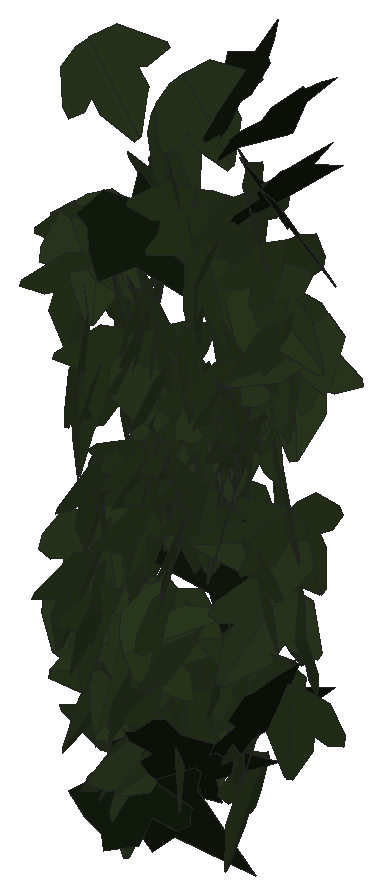
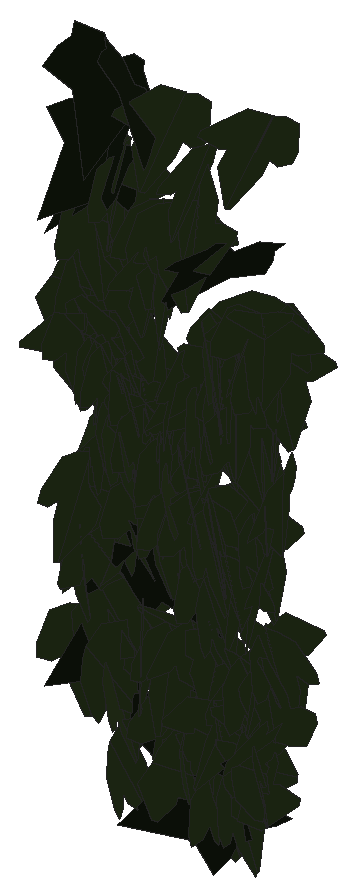
# SketchUp Ruby script. Lengths in inches.
U = 1.inch
M = Sketchup.active_model
def pt(a) = Geom::Point3d.new(a.map { |v| v * U })
def face(e, loops, mat)
  f = e.add_face(loops[0].map { |a| pt(a) })
  loops[1..].each { |l| e.add_face(l.map { |a| pt(a) }).erase! }
  f.material = f.back_material = mat if mat
  f
end
# faces: each face lists its corners as indices into pts; further lists are holes
def faces(e, pts, list, mat = nil) = list.each { |f| face(e, (f[0].is_a?(Array) ? f : [f]).map { |l| l.map { |i| pts[i] } }, mat) }
# xy, xz, yz: faces in a plane at the given z, y or x. An outline is a flat list of corners, or four numbers for a rectangle; further outlines are holes
def ring(l) = l.size == 4 ? [[l[0], l[1]], [l[2], l[1]], [l[2], l[3]], [l[0], l[3]]] : l.each_slice(2).to_a
def flat(e, list, mat, &to3) = list.each { |f| face(e, (f[0].is_a?(Array) ? f : [f]).map { |l| ring(l).map { |u, v| to3.(u, v) } }, mat) }
def xy(e, z, list, mat = nil) = flat(e, list, mat) { |x, y| [x, y, z] }
def xz(e, y, list, mat = nil) = flat(e, list, mat) { |x, z| [x, y, z] }
def yz(e, x, list, mat = nil) = flat(e, list, mat) { |y, z| [x, y, z] }
def lines(e, pts, list) = list.each { |a, b| e.add_line(pt(pts[a]), pt(pts[b])) }
# prism: a flat outline (further loops are holes) pulled along v
def prism(e, loops, v, mat = nil)
  f = face(e, loops, mat); d = Geom::Vector3d.new(v.map { |x| x * U })
  f.pushpull(f.normal.samedirection?(d) ? d.length : -d.length)
end
def box(e, o, s, mat = nil) = prism(e, [[o, [o[0] + s[0], o[1], o[2]], [o[0] + s[0], o[1] + s[1], o[2]], [o[0], o[1] + s[1], o[2]]]], [0, 0, s[2]], mat)
def at(x, y, z, deg = 0) = Geom::Transformation.translation(pt([x, y, z])) * Geom::Transformation.rotation(ORIGIN, Z_AXIS, deg.degrees)
def axes(o, x, y, z) = Geom::Transformation.new([*x, 0, *y, 0, *z, 0, *pt(o).to_a, 1])
def part(name) = M.definitions.add(name)
# library, detail: a bought-in or finely detailed component or shape, given as its bounding box
def library(name, o, s) = part(name).tap { |d| box(d.entities, o, s) }
def detail(e, o, s) = box(e.add_group.entities, o, s)
def put(e, d, t, mat = nil) = e.add_instance(d, t).tap { |i| i.material = mat if mat }
def group(e, t, mat = nil) = e.add_group.tap { |g| g.transformation = t; g.material = mat if mat }.entities
root = M.entities
M.materials.add("efeu1").color = [18, 25, 13]
M.materials.add("efeu2").color = [43, 57, 29]
c1 = part("ivyleaf_10")
p = [[0,0.5,-0.03],[-0.0625,2.02,-0.43],[-0.19,2.01,-0.46],[-0.54,1.05,-0.29],[-0.52,0.625,-0.18],[-0.83,0.76,-0.28],
  [-1.16,0.64,-0.33],[-1.15,0.33,-0.24],[-0.77,-0.39,0.02],[-0.3,-0.51,0.16],[0.04,-0.48,0.23],[-0.02,2.01,-0.4375],
  [-0.06,2.01,-0.43],[0.04,-0.49,0.23],[0.67,-0.49,0.14],[1.38,0.36,-0.2],[1.375,0.51,-0.24],[0.81,0.65,-0.19],
  [0.62,0.59,-0.15],[0.6,1.09,-0.28],[0.5,1.23,-0.31]]
faces(c1.entities,p,[[0,1,2,3,4,5,6,7,8,9,10],[11,12,0,13,14,15,16,17,18,19,20]],"efeu2")
c2 = part("ivyleaf_9")
p = [[1.54,2.16,1.25],[1.36,2.04,1.19],[-0.21,0.99,0.68],[-0.71,1.11,0.82],[-0.85,0.86,0.67],[-0.8,0.17,0.21],
  [-0.9,-0.01,0.1],[-0.67,-0.16,-0.02],[-0.08,-0.08,-0.05],[-0.03,-0.6,-0.4],[0.65,-0.88,-0.66],[0.83,-0.6,-0.49],
  [1.29,-0.42,-0.43],[1.8125,-0.07,-0.26],[1.21,0.44,0.15]]
faces(c2.entities,p,[[0,1,2,3,4,5,6,7,8,9,10,11,12,13,14]],"efeu1")
put(root,c1,axes([27.76,224.9,217.875],[0.32186,-0.37476,0.07721],[0.0469,-0.06149,-0.49398],[0.37975,0.32523,-0.00443]))
put(root,c1,axes([28.11,224.8,221.44],[-0.12731,-0.48235,-0.0336],[0.01522,0.03073,-0.49882],[0.48328,-0.12803,0.00686]))
put(root,c1,axes([27,224.88,220.98],[-0.45625,0.14667,0.14255],[0.12489,-0.0762,0.47812],[0.16197,0.47189,0.0329]))
put(root,c1,axes([27.65,224.8,218.9],[-0.48631,-0.11147,0.03275],[-0.01817,-0.06626,-0.49526],[0.11475,-0.48289,0.06039]))
put(root,c1,axes([26.05,224.64,219.4],[0.22603,-0.33922,-0.28955],[-0.06525,0.29596,-0.39768],[0.44119,0.21756,0.08952]))
put(root,c1,axes([26.27,224.625,222.59],[0.23053,0.39163,0.20853],[0.05646,0.20719,-0.45154],[-0.44008,0.23174,0.05131]))
put(root,c1,axes([26.78,224.75,219.79],[-0.43148,0.24494,-0.0619],[0.04889,-0.03924,-0.49605],[-0.24787,-0.43412,0.00992]))
put(root,c1,axes([27.88,224.69,219.13],[-0.44021,0.19722,0.13159],[-0.12185,0.04985,-0.48235],[-0.20338,-0.45675,0.00417]))
put(root,c2,axes([26.63,224.75,220.96],[0.11537,-0.37052,-0.31528],[0.09739,0.33505,-0.35813],[0.47666,0.02122,0.14948]))
put(root,c1,axes([26.12,224.875,217.59],[0.03942,-0.49822,0.01477],[-0.001,-0.0149,-0.49978],[0.49844,0.03937,-0.00217]))
put(root,c1,axes([26.59,225,214.24],[-0.12687,-0.45195,0.17217],[0.08725,-0.19647,-0.45143],[0.4757,-0.0845,0.12872]))
put(root,c1,axes([27.57,224.8125,221.0625],[-0.2853,-0.4062,-0.06001],[0.07845,0.0178,-0.49349],[0.40305,-0.291,0.05358]))
put(root,c1,axes([28.67,225.06,220.06],[0.1758,0.19948,-0.42344],[-0.3113,-0.28796,-0.2649],[-0.34955,0.35677,0.02295]))
put(root,c1,axes([25.92,224.91,219.86],[-0.25461,-0.41696,0.10639],[-0.0479,-0.09539,-0.48847],[0.42765,-0.25893,0.00863]))
put(root,c2,axes([26.96,224.72,214.59],[0.29944,0.22544,-0.33092],[0.26768,0.19461,0.3748],[0.29779,-0.40163,-0.00414]))
put(root,c1,axes([26.77,224.86,219.67],[0.15933,-0.47141,-0.04881],[-0.00204,0.05082,-0.49741],[0.47393,0.15871,0.01427]))
put(root,c1,axes([25.83,224.96,216.3125],[-0.01159,-0.48963,0.10065],[-0.01001,-0.10043,-0.48971],[0.49977,-0.01337,-0.00747]))
put(root,c1,axes([28.21,224.92,215.95],[-0.35874,-0.19812,0.28645],[-0.23915,-0.15883,-0.40936],[0.2532,-0.43072,0.0192]))
put(root,c1,axes([26.25,224.9,215.59],[0.48382,-0.12583,0.00893],[0.00832,-0.00348,-0.49992],[0.12587,0.48389,-0.00127]))
put(root,c1,axes([27.33,224.87,221.14],[-0.4268,-0.24203,0.09624],[-0.06571,-0.07872,-0.48937],[0.25204,-0.43038,0.03538]))
put(root,c1,axes([28.3125,224.92,216.72],[0.33343,0.27819,-0.24787],[-0.233,-0.10389,-0.43002],[-0.29075,0.40227,0.06036]))
put(root,c1,axes([28.45,224.9,220.91],[-0.19348,-0.46019,0.02807],[0.01283,-0.0358,-0.49855],[0.46087,-0.1922,0.02567]))
put(root,c1,axes([26.71,224.9,218.8],[0.30583,-0.03388,0.39411],[0.39529,0.00756,-0.30609],[0.01478,0.49879,0.03141]))
put(root,c1,axes([28.24,224.68,221.57],[-0.2867,0.36522,0.18552],[-0.14239,0.12348,-0.46312],[-0.3841,-0.31838,0.0332]))
put(root,c1,axes([28.24,224.81,220.44],[0.28634,0.09797,0.39801],[0.38316,0.1085,-0.30236],[-0.14561,0.47815,-0.01294]))
put(root,c2,axes([28.27,224.44,215.53],[0.17365,0.29767,0.36227],[0.16977,0.32019,-0.34447],[-0.43706,0.24264,0.01013]))
put(root,c1,axes([28.55,224.82,220.08],[-0.11985,-0.47617,-0.0943],[0.03761,0.08773,-0.4908],[0.48396,-0.12474,0.01479]))
put(root,c1,axes([27.95,224.87,219.72],[-0.39698,0.06214,-0.29757],[0.2846,-0.09601,-0.39973],[-0.10682,-0.48674,0.04086]))
put(root,c1,axes([26.8,224.75,215.83],[0.24577,-0.06021,-0.43124],[0.43309,0.08507,0.23495],[0.04508,-0.48902,0.09397]))
put(root,c2,axes([28.1875,224.79,221.81],[0.45684,-0.18155,-0.09128],[-0.08373,0.03647,-0.49159],[0.18515,0.46445,0.00291]))
put(root,c1,axes([26.62,224.97,219.1],[0.1077,-0.48462,0.05952],[0.02434,-0.05555,-0.49631],[0.48766,0.1098,0.01163]))
put(root,c1,axes([26.36,224.98,214.29],[0.05304,-0.49244,0.06846],[0.01417,-0.06732,-0.49524],[0.49698,0.05448,0.00682]))
put(root,c1,axes([28.42,224.96,217.51],[0.11904,0.03073,-0.48465],[-0.48181,-0.05495,-0.12182],[-0.06075,0.49602,0.01653]))
put(root,c1,axes([27.11,224.91,217.27],[0.22328,-0.44427,-0.05263],[-0.02908,0.04428,-0.49719],[0.44643,0.22508,-0.00606]))
put(root,c1,axes([25.92,224.9,220.45],[-0.37661,-0.1667,-0.2835],[0.31762,-0.07254,-0.37928],[0.08533,-0.46578,0.16053]))
put(root,c1,axes([27.66,224.58,220.39],[-0.04606,0.26392,0.42217],[-0.31505,0.31284,-0.22994],[-0.38552,-0.28719,0.13748]))
put(root,c2,axes([26.83,224.76,213.85],[-0.49327,-0.06522,0.04932],[0.04903,0.00549,0.49756],[-0.06544,0.4957,0.00098]))
put(root,c1,axes([27.625,224.78,220.59],[0.04077,0.49217,0.07813],[-0.03385,0.08094,-0.49224],[-0.49718,0.03485,0.03992]))
put(root,c1,axes([26.09,225.09,215.91],[-0.06239,-0.46204,0.18064],[0.03324,-0.18555,-0.46311],[0.49498,-0.04578,0.05387]))
put(root,c2,axes([28.47,224.58,222.67],[0.09332,0.47646,0.11949],[-0.01587,0.12449,-0.48399],[-0.49096,0.08654,0.03835]))
put(root,c1,axes([26.34,224.85,219.95],[-0.25046,0.43242,-0.01664],[-0.00683,-0.02317,-0.49942],[-0.43269,-0.24994,0.01752]))
put(root,c1,axes([26.91,225.2,214.72],[0.0959,-0.20544,0.44564],[0.34429,-0.29539,-0.21027],[0.34967,0.34719,0.08481]))
put(root,c1,axes([28.19,224.93,219.47],[-0.4104,0.16587,0.2325],[-0.2745,-0.11666,-0.4013],[-0.07887,-0.45703,0.18682]))
put(root,c1,axes([28.23,225.11,218.21],[0.16858,-0.24164,0.40397],[0.39421,-0.16204,-0.26143],[0.25726,0.40664,0.13588]))
put(root,c1,axes([28.02,224.9,217.2],[-0.40692,0.26497,-0.1192],[0.09256,-0.07623,-0.48541],[-0.27541,-0.41711,0.01299]))
put(root,c1,axes([26.98,224.98,216.14],[0.09407,0.46893,-0.14579],[-0.07354,-0.13331,-0.47626],[-0.48553,0.11105,0.04389]))
put(root,c1,axes([26.12,224.6875,216.05],[0.05681,-0.33327,-0.36838],[-0.02077,0.36887,-0.33691],[0.49633,0.05358,0.02806]))
put(root,c1,axes([26.8,224.62,219.16],[0.15487,0.13747,0.4551],[0.18979,0.42097,-0.19175],[-0.43588,0.23214,0.07821]))
put(root,c1,axes([26.96,225.08,217.12],[0.31368,-0.37447,0.10665],[0.06027,-0.0886,-0.48838],[0.38467,0.31925,-0.01044]))
put(root,c1,axes([26.25,225.04,219.03],[-0.26554,-0.4056,0.12237],[-0.04965,-0.11364,-0.48438],[0.42074,-0.2694,0.02007]))
put(root,c1,axes([25.98,224.95,220.34],[0.42156,0.26885,-0.00194],[-0.00543,0.00491,-0.49995],[-0.2688,0.42154,0.00706]))
put(root,c1,axes([27.73,224.93,218.86],[0.47368,0.14765,0.06182],[0.0449,0.06277,-0.49401],[-0.15365,0.47356,0.04621]))
put(root,c1,axes([27.04,224.8,222.02],[-0.07534,0.48071,0.11507],[-0.01046,0.11482,-0.48652],[-0.49418,-0.07572,-0.00725]))
put(root,c1,axes([27.41,224.75,222.52],[0.22002,0.39021,0.2221],[0.01019,0.24293,-0.4369],[-0.44887,0.19678,0.09895]))
put(root,c1,axes([26.73,224.84,219.74],[0.32683,-0.26541,-0.2697],[-0.13054,0.25542,-0.40954],[0.35516,0.33811,0.09767]))
put(root,c1,axes([27.94,224.95,219.35],[-0.28362,-0.40912,-0.04673],[0.01798,0.04438,-0.4977],[0.41138,-0.284,-0.01047]))
put(root,c1,axes([26.9,224.94,218.97],[0.0918,-0.47177,-0.13785],[-0.02177,0.13619,-0.4806],[0.49102,0.09424,0.00446]))
put(root,c1,axes([25.91,225.33,214.94],[0.0727,-0.2362,0.43466],[0.11784,-0.41841,-0.24708],[0.48045,0.13837,-0.00517]))
put(root,c1,axes([27.6,224.93,218.68],[-0.38445,0.31856,0.02684],[-0.06863,-0.04124,-0.49355],[-0.31223,-0.38317,0.07544]))
put(root,c1,axes([27.28,225.05,218.27],[-0.12694,-0.48284,0.02741],[0.01094,-0.0312,-0.49891],[0.48349,-0.12606,0.01849]))
put(root,c1,axes([25.99,224.98,220.39],[-0.43279,-0.2493,0.02324],[-0.01981,-0.01217,-0.49946],[0.2496,-0.43324,0.00066]))
put(root,c1,axes([27.27,224.83,219.32],[-0.19919,0.43356,0.1495],[-0.10485,0.11562,-0.47501],[-0.44646,-0.22058,0.04486]))
put(root,c2,axes([26.71,224.92,214.09],[0.01321,0.02582,-0.49916],[0.40775,0.28823,0.0257],[0.28907,-0.40775,-0.01344]))
put(root,c1,axes([27.98,225.09,215.23],[0.1511,-0.47578,0.0284],[0.00354,-0.02867,-0.49916],[0.47661,0.15105,-0.0053]))
put(root,c1,axes([28.55,224.99,215.64],[-0.48413,-0.0691,0.10413],[-0.09767,-0.05067,-0.48774],[0.07796,-0.4926,0.03557]))
put(root,c1,axes([27.86,225.1,219.06],[0.32474,-0.37264,0.07539],[0.07691,-0.03271,-0.49297],[0.37233,0.33176,0.03607]))
put(root,c1,axes([26.58,225,219.76],[0.18475,-0.45853,-0.07494],[0.03295,0.09338,-0.4901],[0.46345,0.17615,0.06472]))
put(root,c1,axes([28.02,225.09,218.66],[0.07869,-0.49302,0.02713],[-0.01064,-0.02915,-0.49904],[0.49365,0.07796,-0.01508]))
put(root,c1,axes([28.85,224.8,216.59],[-0.20117,0.14603,0.43383],[-0.39758,0.17911,-0.24465],[-0.22686,-0.44339,0.04406]))
put(root,c1,axes([26.17,225.0625,214.34],[-0.49722,0.03466,-0.03959],[-0.04017,-0.0071,0.49833],[0.03399,0.49875,0.00984]))
put(root,c1,axes([25.7,225.04,218.4375],[-0.10538,0.47666,-0.10814],[-0.03555,-0.11781,-0.48462],[-0.48747,-0.09445,0.05871]))
put(root,c1,axes([27.37,225.06,218.07],[-0.03002,-0.49793,-0.03417],[0.00735,0.03379,-0.4988],[0.49904,-0.03045,0.00529]))
put(root,c1,axes([27.25,224.99,215.86],[-0.17578,-0.45107,-0.12504],[0.0556,0.1125,-0.484],[0.46477,-0.18406,0.0106]))
put(root,c1,axes([27.78,225.07,219.125],[0.01409,-0.49813,-0.04082],[-0.00462,0.0407,-0.49832],[0.49978,0.01442,-0.00345]))
put(root,c1,axes([27.77,225.28,214.39],[0.1179,-0.41651,0.25024],[0.12162,-0.224,-0.43015],[0.47043,0.1623,0.04849]))
put(root,c1,axes([27.36,225.16,218.51],[-0.35576,0.19609,-0.29152],[0.19422,-0.23595,-0.39574],[-0.29277,-0.39481,0.09171]))
put(root,c1,axes([28.16,225.11,219.3],[-0.06078,-0.49625,0.00645],[0.00116,-0.00664,-0.49995],[0.49629,-0.06076,0.00195]))
put(root,c1,axes([27.69,224.92,215.96],[0.17437,-0.39533,-0.25162],[-0.03075,0.25825,-0.42704],[0.4676,0.1644,0.06575]))
put(root,c1,axes([27.3,225.02,218.51],[-0.49507,0.06694,0.02049],[-0.02589,-0.03912,-0.49779],[-0.06504,-0.49395,0.0422]))
put(root,c1,axes([27.52,225.11,217.7],[-0.40525,-0.27323,0.10541],[-0.05929,-0.0997,-0.48636],[0.2868,-0.4067,0.04841]))
put(root,c1,axes([26.8,224.875,217.94],[-0.21054,0.42223,0.16552],[-0.09142,0.13923,-0.47144],[-0.4442,-0.22878,0.01858]))
put(root,c1,axes([27.33,225.11,217.63],[-0.00751,-0.49994,-0.00112],[0.00555,0.00104,-0.49997],[0.49991,-0.00752,0.00553]))
put(root,c1,axes([26.68,225.06,219.93],[0.23756,-0.42799,-0.10192],[-0.0339,0.09768,-0.48919],[0.43865,0.23934,0.01739]))
put(root,c1,axes([28.3,225.1,219.29],[0.399,-0.28691,-0.09208],[-0.08046,0.04581,-0.49135],[0.29039,0.40692,-0.00962]))
put(root,c1,axes([27.86,225.26,218.65],[0.07097,-0.45511,0.19451],[0.02277,-0.19329,-0.46057],[0.49441,0.07423,-0.00671]))
put(root,c1,axes([26.64,225.01,217.74],[0.32715,0.17625,-0.33453],[-0.37668,0.11342,-0.30862],[-0.0329,0.45395,0.20699]))
put(root,c1,axes([27.68,225.18,218.59],[0.1502,-0.47289,0.06175],[0.02899,-0.05557,-0.49606],[0.47602,0.1526,0.01072]))
put(root,c2,axes([28.4,224.66,221.71],[0.19686,0.34637,0.30212],[0.07386,0.30055,-0.3927],[-0.45364,0.19924,0.06717]))
put(root,c1,axes([27.09,225.03,215.07],[-0.42529,-0.25816,-0.04984],[0.04161,0.0275,-0.49751],[0.25961,-0.42731,-0.00191]))
put(root,c1,axes([26.29,225.15,217.24],[0.4864,-0.10053,0.05753],[0.05451,-0.02046,-0.4966],[0.1022,0.48936,-0.00895]))
put(root,c1,axes([25.91,225.42,214.98],[-0.1516,0.17275,0.44405],[0.02226,-0.4629,0.18768],[0.47594,0.07667,0.13266]))
put(root,c1,axes([27.02,225.33,214.5625],[0.14429,0.22157,-0.42437],[-0.30283,-0.30103,-0.26014],[-0.37078,0.33209,0.04732]))
put(root,c1,axes([28.01,225.35,215.56],[0.06148,-0.40446,0.28745],[0.06463,-0.28066,-0.40872],[0.49198,0.08742,0.01777]))
put(root,c1,axes([26.38,225.04,219.41],[-0.47082,0.1121,0.12556],[-0.13266,-0.01757,-0.48176],[-0.1036,-0.48695,0.04629]))
put(root,c1,axes([26.07,225.125,215.125],[0.3295,-0.37022,-0.06613],[-0.03226,0.05978,-0.49536],[0.37469,0.33071,0.01551]))
put(root,c1,axes([28.4,225.09,219.65],[-0.24703,-0.43332,-0.03483],[0.02071,0.02828,-0.49877],[0.43422,-0.24786,0.00397]))
put(root,c1,axes([26.48,225.13,216.03],[0.46326,0.05071,0.18116],[0.17976,0.0227,-0.46602],[-0.05549,0.4969,0.0028]))
put(root,c1,axes([25.69,225.16,216.5],[0.49031,-0.09697,-0.01388],[-0.01349,0.00335,-0.49981],[0.09703,0.4905,0.00067]))
put(root,c1,axes([26.91,225.18,218.36],[0.26851,-0.42115,0.02302],[0.04192,-0.00051,-0.49824],[0.41969,0.2695,0.03504]))
put(root,c1,axes([25.9375,224.97,218.64],[0.15769,-0.38821,-0.27282],[-0.0844,0.25996,-0.41869],[0.46692,0.1781,0.01645]))
put(root,c1,axes([28.45,225.1,219.54],[0.33608,0.37005,0.01065],[-0.00149,0.01574,-0.49975],[-0.3702,0.33588,0.01169]))
put(root,c1,axes([27.01,225.24,218.12],[0.15292,-0.47019,0.07439],[0.01091,-0.07465,-0.49427],[0.47592,0.15279,-0.01257]))
put(root,c2,axes([27.97,224.8,222.65],[-0.0892,0.36118,0.33405],[-0.11884,0.31363,-0.37083],[-0.47741,-0.14555,0.02989]))
put(root,c1,axes([28.4,225.17,219.67],[-0.35957,0.12222,0.32523],[-0.34655,-0.15963,-0.32315],[0.02484,-0.4578,0.19951]))
put(root,c1,axes([26.57,225.17,217.0625],[-0.16037,-0.47329,0.01669],[-0.00955,-0.01438,-0.4997],[0.47349,-0.16059,-0.00443]))
put(root,c1,axes([26.79,225.1,217.76],[0.49665,-0.0146,0.05594],[0.05778,0.10929,-0.48448],[0.00192,0.48769,0.11024]))
put(root,c1,axes([27.44,225.18,218.67],[-0.18287,-0.46457,0.02714],[0.00844,-0.03247,-0.49887],[0.46528,-0.182,0.01972]))
put(root,c1,axes([27.875,225.12,218.67],[0.456,-0.08411,-0.18704],[-0.17134,0.09437,-0.46015],[0.11271,0.48376,0.05724]))
put(root,c1,axes([26.48,225.15,214.83],[0.47021,0.13642,0.10145],[0.09815,0.02581,-0.48959],[-0.13882,0.48034,-0.0025]))
put(root,c1,axes([26.56,225.14,217.91],[0.29117,-0.39851,-0.08003],[-0.01241,0.08969,-0.49173],[0.40628,0.28835,0.04234]))
put(root,c1,axes([27.98,225.15,219.28],[-0.06565,-0.49261,-0.05497],[0.06637,0.04621,-0.49342],[0.49121,-0.07208,0.05932]))
put(root,c1,axes([25.8,225.05,215.35],[0.4667,0.17421,-0.04297],[0.03943,0.01724,0.49814],[0.17504,-0.46835,0.00236]))
put(root,c1,axes([26.56,225.2,217.68],[0.06514,-0.49574,-0.00182],[-0.0112,0.00037,-0.49987],[0.49561,0.06516,-0.01106]))
put(root,c1,axes([25.96,225.01,217.3125],[-0.25263,0.41901,0.10301],[-0.0729,0.07621,-0.48875],[-0.42528,-0.26197,0.02259]))
put(root,c1,axes([26.72,225.15,217.84],[-0.2356,-0.43902,-0.04184],[0.025,0.03406,-0.49821],[0.4403,-0.23685,0.0059]))
put(root,c1,axes([28.4375,225.07,217.65],[-0.18652,-0.42748,-0.1802],[0.12761,0.13945,-0.46289],[0.44601,-0.21867,0.05707]))
put(root,c1,axes([27.86,225,218.58],[0.30657,-0.23523,-0.3173],[-0.16177,0.29166,-0.37251],[0.36035,0.33106,0.10272]))
put(root,c1,axes([26.42,225.21,215.37],[0.44836,0.22016,-0.02237],[-0.01964,-0.01077,-0.4995],[-0.22042,0.44879,-0.00101]))
put(root,c1,axes([27.88,224.89,219.04],[-0.09294,0.36702,0.32659],[-0.15698,0.29277,-0.37369],[-0.46553,-0.172,0.06081]))
put(root,c1,axes([26.41,225.34,216.91],[0.09484,-0.46928,0.14415],[0.07502,-0.13124,-0.4766],[0.48516,0.11202,0.04551]))
put(root,c1,axes([26.63,225.24,217.88],[-0.27481,-0.41549,0.04298],[0.01837,-0.06342,-0.49562],[0.41731,-0.27082,0.05012]))
put(root,c1,axes([26.49,224.9,215.26],[-0.02031,-0.30078,-0.3989],[0.03796,0.39715,-0.30139],[0.49814,-0.04253,0.0067]))
put(root,c1,axes([26.98,225.18,217.76],[-0.22943,-0.44188,-0.04586],[0.04654,0.02742,-0.49707],[0.44181,-0.23236,0.02855]))
put(root,c1,axes([27.76,225.29,218.55],[0.0846,-0.48998,0.05257],[-0.00224,-0.05372,-0.4971],[0.49279,0.08387,-0.01129]))
put(root,c2,axes([27.65,225.18,217.01],[-0.08273,-0.04175,-0.49134],[-0.45745,-0.1795,0.09227],[-0.1841,0.4648,-0.00849]))
put(root,c1,axes([27.0625,224.91,218.125],[-0.19475,0.34093,0.30958],[-0.14858,0.27163,-0.39261],[-0.43589,-0.24491,-0.00449]))
